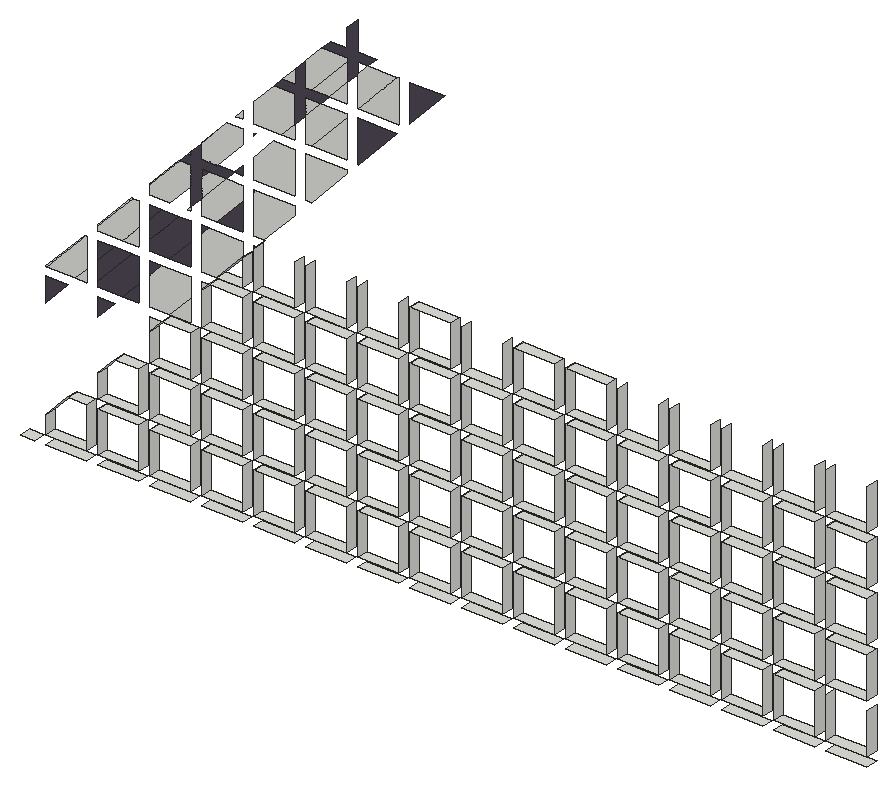
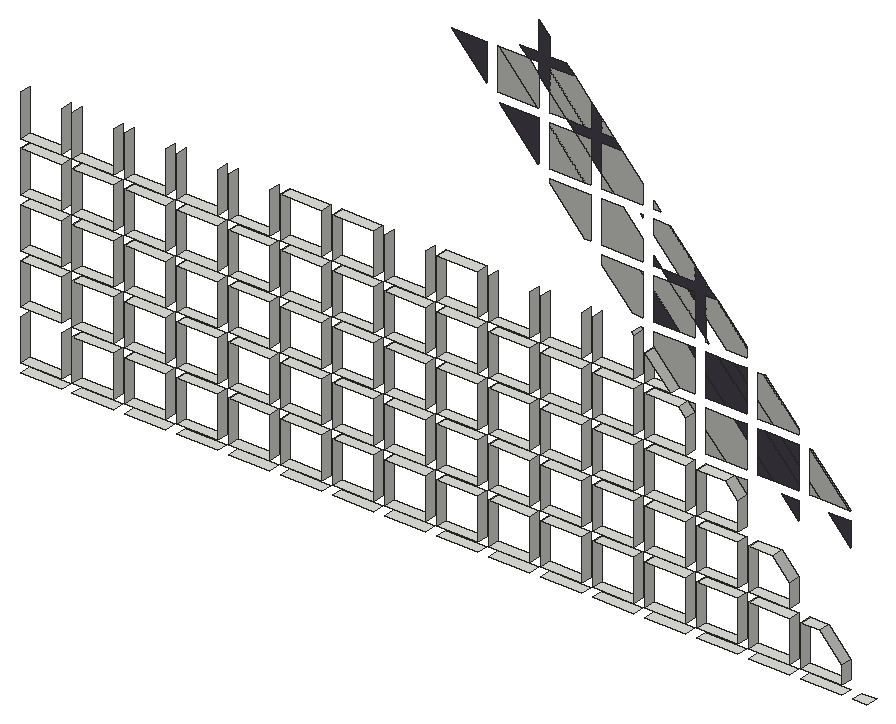
# SketchUp Ruby script. Lengths in inches.
U = 1.inch
M = Sketchup.active_model
def pt(a) = Geom::Point3d.new(a.map { |v| v * U })
def face(e, loops, mat)
  f = e.add_face(loops[0].map { |a| pt(a) })
  loops[1..].each { |l| e.add_face(l.map { |a| pt(a) }).erase! }
  f.material = f.back_material = mat if mat
  f
end
# faces: each face lists its corners as indices into pts; further lists are holes
def faces(e, pts, list, mat = nil) = list.each { |f| face(e, (f[0].is_a?(Array) ? f : [f]).map { |l| l.map { |i| pts[i] } }, mat) }
# xy, xz, yz: faces in a plane at the given z, y or x. An outline is a flat list of corners, or four numbers for a rectangle; further outlines are holes
def ring(l) = l.size == 4 ? [[l[0], l[1]], [l[2], l[1]], [l[2], l[3]], [l[0], l[3]]] : l.each_slice(2).to_a
def flat(e, list, mat, &to3) = list.each { |f| face(e, (f[0].is_a?(Array) ? f : [f]).map { |l| ring(l).map { |u, v| to3.(u, v) } }, mat) }
def xy(e, z, list, mat = nil) = flat(e, list, mat) { |x, y| [x, y, z] }
def xz(e, y, list, mat = nil) = flat(e, list, mat) { |x, z| [x, y, z] }
def yz(e, x, list, mat = nil) = flat(e, list, mat) { |y, z| [x, y, z] }
def lines(e, pts, list) = list.each { |a, b| e.add_line(pt(pts[a]), pt(pts[b])) }
# prism: a flat outline (further loops are holes) pulled along v
def prism(e, loops, v, mat = nil)
  f = face(e, loops, mat); d = Geom::Vector3d.new(v.map { |x| x * U })
  f.pushpull(f.normal.samedirection?(d) ? d.length : -d.length)
end
def box(e, o, s, mat = nil) = prism(e, [[o, [o[0] + s[0], o[1], o[2]], [o[0] + s[0], o[1] + s[1], o[2]], [o[0], o[1] + s[1], o[2]]]], [0, 0, s[2]], mat)
def at(x, y, z, deg = 0) = Geom::Transformation.translation(pt([x, y, z])) * Geom::Transformation.rotation(ORIGIN, Z_AXIS, deg.degrees)
def axes(o, x, y, z) = Geom::Transformation.new([*x, 0, *y, 0, *z, 0, *pt(o).to_a, 1])
def part(name) = M.definitions.add(name)
# library, detail: a bought-in or finely detailed component or shape, given as its bounding box
def library(name, o, s) = part(name).tap { |d| box(d.entities, o, s) }
def detail(e, o, s) = box(e.add_group.entities, o, s)
def put(e, d, t, mat = nil) = e.add_instance(d, t).tap { |i| i.material = mat if mat }
def group(e, t, mat = nil) = e.add_group.tap { |g| g.transformation = t; g.material = mat if mat }.entities
root = M.entities
M.materials.add("[Color M06]").color = [79, 71, 84]
xy(root,341.65,[[970.91,2332.13,971.71,2332.76],[972.3125,2332.13,974.625,2332.76],[975.23,2332.13,977.54,2332.76],[978.14,2332.13,980.45,2332.76],[981.05,2332.13,983.36,2332.76],
  [983.96,2332.13,986.27,2332.76],[986.875,2332.13,989.1875,2332.76],[989.79,2332.13,992.1,2332.76],[992.7,2332.13,995.01,2332.76],[995.61,2332.13,997.92,2332.76],
  [998.52,2332.13,1000.83,2332.76],[1001.43,2332.13,1003.75,2332.76],[1004.35,2332.13,1006.66,2332.76],[1007.26,2332.13,1009.57,2332.76],[1010.17,2332.13,1012.48,2332.76],
  [1013.08,2332.13,1015.4,2332.76],[1015.99,2332.13,1018.31,2332.76]])
xy(root,342.15,[[972.3125,2332.13,974.625,2332.76],[975.23,2332.13,977.54,2332.76],[978.14,2332.13,980.45,2332.76],[981.05,2332.13,983.36,2332.76],[983.96,2332.13,986.27,2332.76],
  [986.875,2332.13,989.1875,2332.76],[989.79,2332.13,992.1,2332.76],[992.7,2332.13,995.01,2332.76],[995.61,2332.13,997.92,2332.76],[998.52,2332.13,1000.83,2332.76],
  [1001.43,2332.13,1003.75,2332.76],[1004.35,2332.13,1006.66,2332.76],[1007.26,2332.13,1009.57,2332.76],[1010.17,2332.13,1012.48,2332.76],[1013.08,2332.13,1015.4,2332.76],
  [1015.99,2332.13,1018.31,2332.76]])
xy(root,344.46,[[973.55,2332.13,974.625,2332.76],[975.23,2332.13,977.54,2332.76],[978.14,2332.13,980.45,2332.76],[981.05,2332.13,983.36,2332.76],[983.96,2332.13,986.27,2332.76],
  [986.875,2332.13,989.1875,2332.76],[989.79,2332.13,992.1,2332.76],[992.7,2332.13,995.01,2332.76],[995.61,2332.13,997.92,2332.76],[998.52,2332.13,1000.83,2332.76],
  [1001.43,2332.13,1003.75,2332.76],[1004.35,2332.13,1006.66,2332.76],[1007.26,2332.13,1009.57,2332.76],[1010.17,2332.13,1012.48,2332.76],[1013.08,2332.13,1015.4,2332.76]])
xy(root,344.96,[[975.23,2332.13,977.54,2332.76],[978.14,2332.13,980.45,2332.76],[981.05,2332.13,983.36,2332.76],[983.96,2332.13,986.27,2332.76],[986.875,2332.13,989.1875,2332.76],
  [989.79,2332.13,992.1,2332.76],[992.7,2332.13,995.01,2332.76],[995.61,2332.13,997.92,2332.76],[998.52,2332.13,1000.83,2332.76],[1001.43,2332.13,1003.75,2332.76],
  [1004.35,2332.13,1006.66,2332.76],[1007.26,2332.13,1009.57,2332.76],[1010.17,2332.13,1012.48,2332.76],[1013.08,2332.13,1015.4,2332.76],[1015.99,2332.13,1018.31,2332.76]])
xy(root,347.27,[[976.1875,2332.13,977.54,2332.76],[978.14,2332.13,980.45,2332.76],[981.05,2332.13,983.36,2332.76],[983.96,2332.13,986.27,2332.76],[986.875,2332.13,989.1875,2332.76],
  [989.79,2332.13,992.1,2332.76],[992.7,2332.13,995.01,2332.76],[995.61,2332.13,997.92,2332.76],[998.52,2332.13,1000.83,2332.76],[1001.43,2332.13,1003.75,2332.76],
  [1004.35,2332.13,1006.66,2332.76],[1007.26,2332.13,1009.57,2332.76],[1010.17,2332.13,1012.48,2332.76],[1013.08,2332.13,1015.4,2332.76],[1015.99,2332.13,1018.31,2332.76]])
xy(root,347.77,[[978.14,2332.13,980.45,2332.76],[981.05,2332.13,983.36,2332.76],[983.96,2332.13,986.27,2332.76],[986.875,2332.13,989.1875,2332.76],[989.79,2332.13,992.1,2332.76],
  [992.7,2332.13,995.01,2332.76],[995.61,2332.13,997.92,2332.76],[998.52,2332.13,1000.83,2332.76],[1001.43,2332.13,1003.75,2332.76],[1004.35,2332.13,1006.66,2332.76],
  [1007.26,2332.13,1009.57,2332.76],[1010.17,2332.13,1012.48,2332.76],[1013.08,2332.13,1015.4,2332.76],[1015.99,2332.13,1018.31,2332.76]])
xy(root,350.09,[[978.82,2332.13,980.45,2332.76],[981.05,2332.13,983.36,2332.76],[983.96,2332.13,986.27,2332.76],[986.875,2332.13,989.1875,2332.76],[989.79,2332.13,992.1,2332.76],
  [992.7,2332.13,995.01,2332.76],[995.61,2332.13,997.92,2332.76],[998.52,2332.13,1000.83,2332.76],[1001.43,2332.13,1003.75,2332.76],[1004.35,2332.13,1006.66,2332.76],
  [1007.26,2332.13,1009.57,2332.76],[1010.17,2332.13,1012.48,2332.76],[1013.08,2332.13,1015.4,2332.76],[1015.99,2332.13,1018.31,2332.76]])
xy(root,350.59,[[981.05,2332.13,983.36,2332.76],[983.96,2332.13,986.27,2332.76],[986.875,2332.13,989.1875,2332.76],[989.79,2332.13,992.1,2332.76],[992.7,2332.13,995.01,2332.76],
  [995.61,2332.13,997.92,2332.76],[998.52,2332.13,1000.83,2332.76],[1001.43,2332.13,1003.75,2332.76],[1004.35,2332.13,1006.66,2332.76],[1007.26,2332.13,1009.57,2332.76],
  [1010.17,2332.13,1012.48,2332.76],[1013.08,2332.13,1015.4,2332.76],[1015.99,2332.13,1018.31,2332.76]])
xy(root,352.9,[[981.46,2332.13,983.36,2332.76],[983.96,2332.13,986.27,2332.76],[986.875,2332.13,989.1875,2332.76],[989.79,2332.13,992.1,2332.76],[992.7,2332.13,995.01,2332.76],
  [995.61,2332.13,997.92,2332.76],[998.52,2332.13,1000.83,2332.76],[1001.43,2332.13,1003.75,2332.76],[1004.35,2332.13,1006.66,2332.76],[1007.26,2332.13,1009.57,2332.76],
  [1010.17,2332.13,1012.48,2332.76],[1013.08,2332.13,1015.4,2332.76],[1015.99,2332.13,1018.31,2332.76]])
xy(root,353.4,[[981.93,2332.13,983.36,2332.76],[983.96,2332.13,986.27,2332.76],[986.875,2332.13,989.1875,2332.76],[989.79,2332.13,992.1,2332.76],[992.7,2332.13,995.01,2332.76],
  [995.61,2332.13,997.92,2332.76],[998.52,2332.13,1000.83,2332.76],[1001.43,2332.13,1003.75,2332.76],[1004.35,2332.13,1006.66,2332.76],[1007.26,2332.13,1009.57,2332.76],
  [1010.17,2332.13,1012.48,2332.76],[1013.08,2332.13,1015.4,2332.76],[1015.99,2332.13,1018.31,2332.76]])
xy(root,355.71,[[992.7,2332.13,995.01,2332.76],[998.52,2332.13,1000.83,2332.76],[1001.43,2332.13,1003.75,2332.76]])
xz(root,2332.13,[[978.14,349.36,978.82,350.09,978.14,350.09],[972.32,350.59,972.375,350.59,974.55,352.9,974.5,352.9],[972.375,350.59,974.02,350.59,974.625,351.24,974.625,352.9,974.55,352.9],[974.02,350.59,974.625,350.59,974.625,351.24],[978.14,350.59,979.29,350.59,980.45,351.82,980.45,352.9,978.82,352.9,978.14,352.17],
  [979.29,350.59,980.45,350.59,980.45,351.82],[981.05,352.46,981.46,352.9,981.05,352.9],[975.23,353.4,976.65,353.4,977.54,354.34,977.54,355.71,977.2,355.71,975.23,353.62],[976.65,353.4,977.54,353.4,977.54,354.34],[981.05,353.4,981.93,353.4,983.36,354.93,983.36,355.71,981.46,355.71,981.05,355.28],
  [975.23,353.62,977.2,355.71,977.15,355.71,975.23,353.67],[983.96,355.57,984.09,355.71,983.96,355.71],[978.14,356.21,979.29,356.21,980.45,357.45,980.45,358.52,979.85,358.52,978.14,356.71],[980.26,356.21,980.45,356.21,980.45,356.41],[981.05,356.21,981.93,356.21,983.36,357.74,983.36,358.52,982.44,358.52,981.05,357.05],
  [983.96,356.21,984.5625,356.21,986.27,358.04,986.27,358.52,984.09,358.52,983.96,358.38],[978.14,356.71,979.85,358.52,979.79,358.52,978.14,356.77],[981.05,357.05,982.44,358.52,981.46,358.52,981.05,358.09],[983.96,358.38,984.09,358.52,983.96,358.52],[980.32,359.02,980.45,359.02,980.45,359.17],
  [981.05,359.02,981.93,359.02,983.36,360.56,983.36,361.34,982.49,361.34,981.05,359.8],[983.96,359.02,986.27,359.02,986.27,361.34,985.09,361.34,983.96,360.14],[986.875,359.02,987.2,359.02,989.1875,361.14,989.1875,361.34,986.875,361.34],[981.05,359.8,982.49,361.34,982.44,361.34,981.05,359.86],[982.97,361.84,983.36,361.84,983.36,362.26],
  [983.96,361.84,985.56,361.84,986.27,362.6,986.27,364.15,985.14,364.15,983.96,362.9],[985.56,361.84,986.27,361.84,986.27,362.6],[986.875,361.84,987.2,361.84,989.1875,363.96,989.1875,364.15,987.74,364.15,986.875,363.23],[987.2,361.84,989.1875,361.84,989.1875,363.96],[986.875,363.23,987.74,364.15,986.875,364.15],
  [985.61,364.65,986.27,364.65,986.27,365.35],[986.875,364.65,987.2,364.65,989.1875,366.77,989.1875,366.96,987.79,366.96,986.875,365.99],[987.2,364.65,988.21,364.65,989.1875,365.69,989.1875,366.77],[988.21,364.65,989.1875,364.65,989.1875,365.69],[989.79,364.65,989.84,364.65,992,366.96,990.38,366.96,989.79,366.33],
  [989.84,364.65,992.1,364.65,992.1,366.96,992,366.96]])
xz(root,2332.13,[[972.3125,348.77,973.55,350.09,972.3125,350.09],[975.23,349.0625,976.1875,350.09,975.23,350.09],[975.23,350.59,976.65,350.59,977.54,351.53,977.54,352.9,977.15,352.9,975.23,350.86],[976.65,350.59,977.54,350.59,977.54,351.53],[975.23,350.86,977.15,352.9,976.1875,352.9,975.23,351.875],
  [975.23,351.875,976.1875,352.9,975.23,352.9],[978.14,352.17,978.82,352.9,978.14,352.9],[978.14,353.4,979.29,353.4,980.45,354.64,980.45,355.71,979.79,355.71,978.14,353.95],[979.29,353.4,980.45,353.4,980.45,354.64],[978.14,353.95,979.79,355.71,978.82,355.71,978.14,354.98],
  [978.14,354.98,978.82,355.71,978.14,355.71],[981.05,355.28,981.46,355.71,981.05,355.71],[981.93,356.21,983.36,356.21,983.36,357.74],[980.45,356.41,981.05,357.05,981.05,358.52,982.44,358.52,982.91,359.02,981.05,359.02,981.05,359.8,980.45,359.17,980.45,359.02,980.32,359.02,979.85,358.52,980.45,358.52],[981.05,358.09,981.46,358.52,981.05,358.52],
  [982.91,359.02,983.36,359.02,983.36,359.5],[983.96,361.2,984.09,361.34,983.96,361.34],[989.79,361.84,989.84,361.84,992,364.15,989.79,364.15],[986.27,362.6,986.875,363.23,986.875,364.15,987.74,364.15,988.21,364.65,986.875,364.65,986.875,365.99,986.27,365.35,986.27,364.65,985.61,364.65,985.14,364.15,986.27,364.15],[992.7,364.89,994.64,366.96,992.7,366.96],
  [989.1875,365.69,989.79,366.33,989.79,366.96,990.38,366.96,990.85,367.46,989.79,367.46,989.79,369.08,989.1875,368.45,989.1875,367.46,988.26,367.46,987.79,366.96,989.1875,366.96]],"[Color M06]")
yz(root,972.3125,[[2332.13,342.15,2332.76,343.14]])
yz(root,974.625,[[2332.13,342.15,2332.76,344.46]])
yz(root,975.23,[[2332.13,342.15,2332.76,344.46],[2332.13,344.96,2332.76,346.25]])
yz(root,977.54,[[2332.13,342.15,2332.76,344.46],[2332.13,344.96,2332.76,347.27]])
yz(root,978.14,[[2332.13,342.15,2332.76,344.46],[2332.13,344.96,2332.76,347.27],[2332.13,347.77,2332.76,349.36]])
yz(root,980.45,[[2332.13,342.15,2332.76,344.46],[2332.13,344.96,2332.76,347.27],[2332.13,347.77,2332.76,350.09]])
yz(root,981.05,[[2332.13,342.15,2332.76,344.46],[2332.13,344.96,2332.76,347.27],[2332.13,347.77,2332.76,350.09],[2332.13,350.59,2332.76,352.46]])
yz(root,983.36,[[2332.13,342.15,2332.76,344.46],[2332.13,344.96,2332.76,347.27],[2332.13,347.77,2332.76,350.09],[2332.13,350.59,2332.76,352.9],[2332.13,353.4,2332.76,354.93]])
yz(root,983.96,[[2332.13,342.15,2332.76,344.46],[2332.13,344.96,2332.76,347.27],[2332.13,347.77,2332.76,350.09],[2332.13,350.59,2332.76,352.9],[2332.13,353.4,2332.76,355.57]])
yz(root,986.27,[[2332.13,342.15,2332.76,344.46],[2332.13,344.96,2332.76,347.27],[2332.13,347.77,2332.76,350.09],[2332.13,350.59,2332.76,352.9],[2332.13,353.4,2332.76,355.71]])
yz(root,986.875,[[2332.13,342.15,2332.76,344.46],[2332.13,344.96,2332.76,347.27],[2332.13,347.77,2332.76,350.09],[2332.13,350.59,2332.76,352.9],[2332.13,353.4,2332.76,355.71]])
yz(root,989.1875,[[2332.13,342.15,2332.76,344.46],[2332.13,344.96,2332.76,347.27],[2332.13,347.77,2332.76,350.09],[2332.13,350.59,2332.76,352.9],[2332.13,353.4,2332.76,355.71]])
yz(root,989.79,[[2332.13,342.15,2332.76,344.46],[2332.13,344.96,2332.76,347.27],[2332.13,347.77,2332.76,350.09],[2332.13,350.59,2332.76,352.9],[2332.13,353.4,2332.76,355.71]])
yz(root,992.1,[[2332.13,342.15,2332.76,344.46],[2332.13,344.96,2332.76,347.27],[2332.13,347.77,2332.76,350.09],[2332.13,350.59,2332.76,352.9],[2332.13,353.4,2332.76,355.71]])
yz(root,992.7,[[2332.13,342.15,2332.76,344.46],[2332.13,344.96,2332.76,347.27],[2332.13,347.77,2332.76,350.09],[2332.13,350.59,2332.76,352.9],[2332.13,353.4,2332.76,355.71]])
yz(root,995.01,[[2332.13,342.15,2332.76,344.46],[2332.13,344.96,2332.76,347.27],[2332.13,347.77,2332.76,350.09],[2332.13,350.59,2332.76,352.9],[2332.13,353.4,2332.76,355.71]])
yz(root,995.61,[[2332.13,342.15,2332.76,344.46],[2332.13,344.96,2332.76,347.27],[2332.13,347.77,2332.76,350.09],[2332.13,350.59,2332.76,352.9],[2332.13,353.4,2332.76,355.71]])
yz(root,997.92,[[2332.13,342.15,2332.76,344.46],[2332.13,344.96,2332.76,347.27],[2332.13,347.77,2332.76,350.09],[2332.13,350.59,2332.76,352.9],[2332.13,353.4,2332.76,355.71]])
yz(root,998.52,[[2332.13,342.15,2332.76,344.46],[2332.13,344.96,2332.76,347.27],[2332.13,347.77,2332.76,350.09],[2332.13,350.59,2332.76,352.9],[2332.13,353.4,2332.76,355.71]])
yz(root,1000.83,[[2332.13,342.15,2332.76,344.46],[2332.13,344.96,2332.76,347.27],[2332.13,347.77,2332.76,350.09],[2332.13,350.59,2332.76,352.9],[2332.13,353.4,2332.76,355.71]])
yz(root,1001.43,[[2332.13,342.15,2332.76,344.46],[2332.13,344.96,2332.76,347.27],[2332.13,347.77,2332.76,350.09],[2332.13,350.59,2332.76,352.9],[2332.13,353.4,2332.76,355.71]])
yz(root,1003.75,[[2332.13,342.15,2332.76,344.46],[2332.13,344.96,2332.76,347.27],[2332.13,347.77,2332.76,350.09],[2332.13,350.59,2332.76,352.9],[2332.13,353.4,2332.76,355.71]])
yz(root,1004.35,[[2332.13,342.15,2332.76,344.46],[2332.13,344.96,2332.76,347.27],[2332.13,347.77,2332.76,350.09],[2332.13,350.59,2332.76,352.9],[2332.13,353.4,2332.76,355.71]])
yz(root,1006.66,[[2332.13,342.15,2332.76,344.46],[2332.13,344.96,2332.76,347.27],[2332.13,347.77,2332.76,350.09],[2332.13,350.59,2332.76,352.9],[2332.13,353.4,2332.76,355.71]])
yz(root,1007.26,[[2332.13,342.15,2332.76,344.46],[2332.13,344.96,2332.76,347.27],[2332.13,347.77,2332.76,350.09],[2332.13,350.59,2332.76,352.9],[2332.13,353.4,2332.76,355.71]])
yz(root,1009.57,[[2332.13,342.15,2332.76,344.46],[2332.13,344.96,2332.76,347.27],[2332.13,347.77,2332.76,350.09],[2332.13,350.59,2332.76,352.9],[2332.13,353.4,2332.76,355.71]])
yz(root,1010.17,[[2332.13,342.15,2332.76,344.46],[2332.13,344.96,2332.76,347.27],[2332.13,347.77,2332.76,350.09],[2332.13,350.59,2332.76,352.9],[2332.13,353.4,2332.76,355.71]])
yz(root,1012.48,[[2332.13,342.15,2332.76,344.46],[2332.13,344.96,2332.76,347.27],[2332.13,347.77,2332.76,350.09],[2332.13,350.59,2332.76,352.9],[2332.13,353.4,2332.76,355.71]])
yz(root,1013.08,[[2332.13,342.15,2332.76,344.46],[2332.13,344.96,2332.76,347.27],[2332.13,347.77,2332.76,350.09],[2332.13,350.59,2332.76,352.9],[2332.13,353.4,2332.76,355.71]])
yz(root,1015.4,[[2332.13,342.15,2332.76,344.46],[2332.13,344.96,2332.76,347.27],[2332.13,347.77,2332.76,350.09],[2332.13,350.59,2332.76,352.9],[2332.13,353.4,2332.76,355.71]])
yz(root,1015.99,[[2332.13,342.15,2332.76,344.46],[2332.13,344.96,2332.76,347.27],[2332.13,347.77,2332.76,350.09],[2332.13,350.59,2332.76,352.9],[2332.13,353.4,2332.76,355.71]])
yz(root,1018.31,[[2332.13,342.15,2332.76,344.46],[2332.13,344.96,2332.76,347.27],[2332.13,347.77,2332.76,350.09],[2332.13,350.59,2332.76,352.9],[2332.13,353.4,2332.76,355.71]])
p = [[973.55,2332.13,344.46],[972.3125,2332.13,343.14],[972.3125,2332.76,343.14],[973.55,2332.76,344.46],[976.1875,2332.13,347.27],[975.23,2332.13,346.25],
  [975.23,2332.76,346.25],[976.1875,2332.76,347.27],[978.82,2332.13,350.09],[978.14,2332.13,349.36],[978.14,2332.76,349.36],[978.82,2332.76,350.09],
  [981.46,2332.13,352.9],[981.05,2332.13,352.46],[981.05,2332.76,352.46],[981.46,2332.76,352.9],[983.36,2332.13,354.93],[981.93,2332.13,353.4],
  [981.93,2332.76,353.4],[983.36,2332.76,354.93],[984.09,2332.13,355.71],[983.96,2332.13,355.57],[983.96,2332.76,355.57],[984.09,2332.76,355.71]]
faces(root,p,[[0,1,2,3],[4,5,6,7],[8,9,10,11],[12,13,14,15],[16,17,18,19],[20,21,22,23]])
